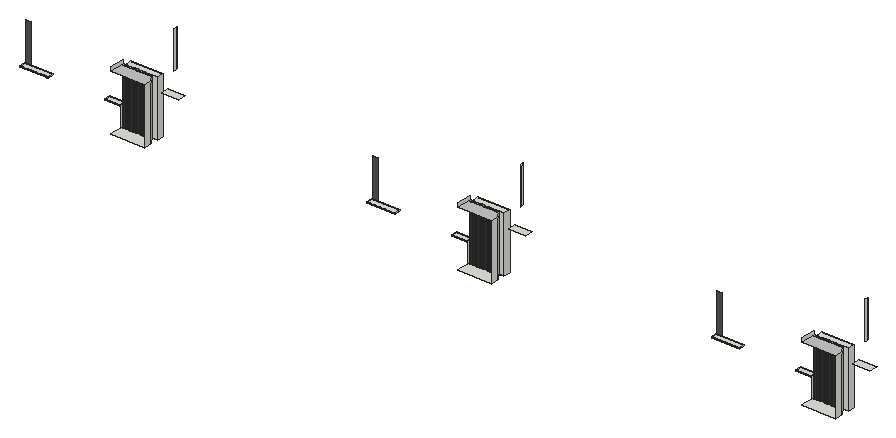
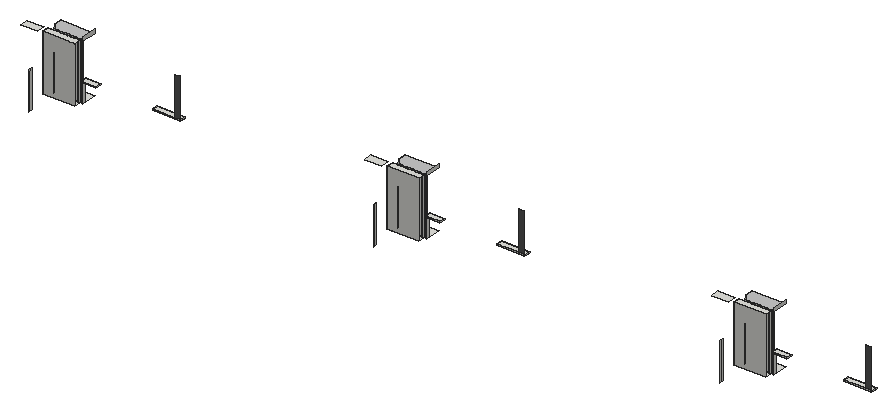
# SketchUp Ruby script. Lengths in inches.
U = 1.inch
M = Sketchup.active_model
def pt(a) = Geom::Point3d.new(a.map { |v| v * U })
def face(e, loops, mat)
  f = e.add_face(loops[0].map { |a| pt(a) })
  loops[1..].each { |l| e.add_face(l.map { |a| pt(a) }).erase! }
  f.material = f.back_material = mat if mat
  f
end
# faces: each face lists its corners as indices into pts; further lists are holes
def faces(e, pts, list, mat = nil) = list.each { |f| face(e, (f[0].is_a?(Array) ? f : [f]).map { |l| l.map { |i| pts[i] } }, mat) }
# xy, xz, yz: faces in a plane at the given z, y or x. An outline is a flat list of corners, or four numbers for a rectangle; further outlines are holes
def ring(l) = l.size == 4 ? [[l[0], l[1]], [l[2], l[1]], [l[2], l[3]], [l[0], l[3]]] : l.each_slice(2).to_a
def flat(e, list, mat, &to3) = list.each { |f| face(e, (f[0].is_a?(Array) ? f : [f]).map { |l| ring(l).map { |u, v| to3.(u, v) } }, mat) }
def xy(e, z, list, mat = nil) = flat(e, list, mat) { |x, y| [x, y, z] }
def xz(e, y, list, mat = nil) = flat(e, list, mat) { |x, z| [x, y, z] }
def yz(e, x, list, mat = nil) = flat(e, list, mat) { |y, z| [x, y, z] }
def lines(e, pts, list) = list.each { |a, b| e.add_line(pt(pts[a]), pt(pts[b])) }
# prism: a flat outline (further loops are holes) pulled along v
def prism(e, loops, v, mat = nil)
  f = face(e, loops, mat); d = Geom::Vector3d.new(v.map { |x| x * U })
  f.pushpull(f.normal.samedirection?(d) ? d.length : -d.length)
end
def box(e, o, s, mat = nil) = prism(e, [[o, [o[0] + s[0], o[1], o[2]], [o[0] + s[0], o[1] + s[1], o[2]], [o[0], o[1] + s[1], o[2]]]], [0, 0, s[2]], mat)
def at(x, y, z, deg = 0) = Geom::Transformation.translation(pt([x, y, z])) * Geom::Transformation.rotation(ORIGIN, Z_AXIS, deg.degrees)
def axes(o, x, y, z) = Geom::Transformation.new([*x, 0, *y, 0, *z, 0, *pt(o).to_a, 1])
def part(name) = M.definitions.add(name)
# library, detail: a bought-in or finely detailed component or shape, given as its bounding box
def library(name, o, s) = part(name).tap { |d| box(d.entities, o, s) }
def detail(e, o, s) = box(e.add_group.entities, o, s)
def put(e, d, t, mat = nil) = e.add_instance(d, t).tap { |i| i.material = mat if mat }
def group(e, t, mat = nil) = e.add_group.tap { |g| g.transformation = t; g.material = mat if mat }.entities
root = M.entities
M.materials.add("[Color M02]").color = [198, 198, 198]
M.materials.add("[Color M06]").color = [86, 86, 86]
M.materials.add("[Color M07]").color = [58, 58, 58]
xy(root,400.68,[[1098.03,273.0625,1175.84,273.0625,1175.84,289.5,1162.46,308.24,1162.46,304.93,1156.61,304.93,1156.61,308.24,1154.46,308.24,1154.46,304.93,1148.61,304.93,1148.61,308.24,1146.46,308.24,1146.46,304.93,1140.61,304.93,1140.61,308.24,1138.46,308.24,1138.46,304.93,1132.61,304.93,1132.61,308.24,1130.46,308.24,1130.46,304.93,1124.61,304.93,1124.61,308.24,1122.46,308.24,1122.46,304.93,1116.61,304.93,1116.61,308.24,1114.46,308.24,1114.46,304.93,1108.61,304.93,1108.61,308.24,1106.46,308.24,1106.46,304.93,1100.61,304.93,1100.61,308.24,1098.03,308.24],[1884.4,273.0625,1962.22,273.0625,1962.22,289.5,1948.83,308.24,1948.83,304.93,1942.98,304.93,1942.98,308.24,1940.83,308.24,1940.83,304.93,1934.98,304.93,1934.98,308.24,1932.83,308.24,1932.83,304.93,1926.98,304.93,1926.98,308.24,1924.83,308.24,1924.83,304.93,1918.98,304.93,1918.98,308.24,1916.83,308.24,1916.83,304.93,1910.98,304.93,1910.98,308.24,1908.83,308.24,1908.83,304.93,1902.98,304.93,1902.98,308.24,1900.83,308.24,1900.83,304.93,1894.98,304.93,1894.98,308.24,1892.83,308.24,1892.83,304.93,1886.98,304.93,1886.98,308.24,1884.4,308.24],[2664.78,273.0625,2742.59,273.0625,2742.59,289.5,2729.21,308.24,2729.21,304.93,2723.36,304.93,2723.36,308.24,2721.21,308.24,2721.21,304.93,2715.36,304.93,2715.36,308.24,2713.21,308.24,2713.21,304.93,2707.36,304.93,2707.36,308.24,2705.21,308.24,2705.21,304.93,2699.36,304.93,2699.36,308.24,2697.21,308.24,2697.21,304.93,2691.36,304.93,2691.36,308.24,2689.21,308.24,2689.21,304.93,2683.36,304.93,2683.36,308.24,2681.21,308.24,2681.21,304.93,2675.36,304.93,2675.36,308.24,2673.21,308.24,2673.21,304.93,2667.36,304.93,2667.36,308.24,2664.78,308.24],[1103.7,304.93,1106.46,308.24],[1108.61,304.93,1114.46,308.24],
  [1116.61,304.93,1122.46,308.24],[1124.61,304.93,1130.46,308.24],[1132.61,304.93,1138.46,308.24],[1140.61,304.93,1146.46,308.24],[1148.61,304.93,1154.46,308.24],
  [1156.61,304.93,1162.46,308.24],[1890.08,304.93,1892.83,308.24],[1894.98,304.93,1900.83,308.24],[1902.98,304.93,1908.83,308.24],[1910.98,304.93,1916.83,308.24],
  [1918.98,304.93,1924.83,308.24],[1926.98,304.93,1932.83,308.24],[1934.98,304.93,1940.83,308.24],[1942.98,304.93,1948.83,308.24],[2670.45,304.93,2673.21,308.24],
  [2675.36,304.93,2681.21,308.24],[2683.36,304.93,2689.21,308.24],[2691.36,304.93,2697.21,308.24],[2699.36,304.93,2705.21,308.24],[2707.36,304.93,2713.21,308.24],
  [2715.36,304.93,2721.21,308.24],[2723.36,304.93,2729.21,308.24],[1103.7,308.24,1175.84,323.81],[1890.08,308.24,1962.22,323.81],[2670.45,308.24,2742.59,323.81]])
xy(root,446.625,[[872.53,298.8125,936.06,301],[1064.56,298.8125,1098.03,301],[1658.9,298.8125,1722.43,301],[1850.93,298.8125,1884.4,301],[2439.28,298.8125,2502.81,301],
  [2631.31,298.8125,2664.78,301],[872.53,301,874.71,311.64],[874.71,301,933.87,311.64],[933.87,301,936.06,311.64],[1064.56,301,1066.62,311.64],
  [1066.62,301,1098.03,311.64],[1658.9,301,1661.09,311.64],[1661.09,301,1720.25,311.64],[1720.25,301,1722.43,311.64],[1850.93,301,1852.99,311.64],
  [1852.99,301,1884.4,311.64],[2439.28,301,2441.46,311.64],[2441.46,301,2500.62,311.64],[2500.62,301,2502.81,311.64],[2631.31,301,2633.37,311.64],
  [2633.37,301,2664.78,311.64]])
xy(root,449.125,[[872.53,298.8125,936.06,311.64],[1064.56,298.8125,1098.03,311.64],[1658.9,298.8125,1722.43,311.64],[1850.93,298.8125,1884.4,311.64],[2439.28,298.8125,2502.81,311.64],
  [2631.31,298.8125,2664.78,311.64]])
xy(root,512.23,[[1200.15,289.5,1239.03,308.24],[1986.53,289.5,2025.4,308.24],[2766.9,289.5,2805.78,308.24]])
xy(root,528.11,[[1103.7,304.93,1106.46,308.24],[1108.61,304.93,1114.46,308.24],[1116.61,304.93,1122.46,308.24],[1124.61,304.93,1130.46,308.24],[1132.61,304.93,1138.46,308.24],
  [1140.61,304.93,1146.46,308.24],[1148.61,304.93,1154.46,308.24],[1156.61,304.93,1162.46,308.24],[1890.08,304.93,1892.83,308.24],[1894.98,304.93,1900.83,308.24],
  [1902.98,304.93,1908.83,308.24],[1910.98,304.93,1916.83,308.24],[1918.98,304.93,1924.83,308.24],[1926.98,304.93,1932.83,308.24],[1934.98,304.93,1940.83,308.24],
  [1942.98,304.93,1948.83,308.24],[2670.45,304.93,2673.21,308.24],[2675.36,304.93,2681.21,308.24],[2683.36,304.93,2689.21,308.24],[2691.36,304.93,2697.21,308.24],
  [2699.36,304.93,2705.21,308.24],[2707.36,304.93,2713.21,308.24],[2715.36,304.93,2721.21,308.24],[2723.36,304.93,2729.21,308.24],[1103.7,308.24,1175.84,323.81],
  [1890.08,308.24,1962.22,323.81],[2670.45,308.24,2742.59,323.81]])
xy(root,528.11,[[1098.03,273.0625,1098.03,308.24,1100.61,308.24,1100.61,304.93,1106.46,304.93,1106.46,308.24,1108.61,308.24,1108.61,304.93,1114.46,304.93,1114.46,308.24,1116.61,308.24,1116.61,304.93,1122.46,304.93,1122.46,308.24,1124.61,308.24,1124.61,304.93,1130.46,304.93,1130.46,308.24,1132.61,308.24,1132.61,304.93,1138.46,304.93,1138.46,308.24,1140.61,308.24,1140.61,304.93,1146.46,304.93,1146.46,308.24,1148.61,308.24,1148.61,304.93,1154.46,304.93,1154.46,308.24,1156.61,308.24,1156.61,304.93,1162.46,304.93,1162.46,308.24,1175.84,289.5,1175.84,273.0625],[1884.4,273.0625,1884.4,308.24,1886.98,308.24,1886.98,304.93,1892.83,304.93,1892.83,308.24,1894.98,308.24,1894.98,304.93,1900.83,304.93,1900.83,308.24,1902.98,308.24,1902.98,304.93,1908.83,304.93,1908.83,308.24,1910.98,308.24,1910.98,304.93,1916.83,304.93,1916.83,308.24,1918.98,308.24,1918.98,304.93,1924.83,304.93,1924.83,308.24,1926.98,308.24,1926.98,304.93,1932.83,304.93,1932.83,308.24,1934.98,308.24,1934.98,304.93,1940.83,304.93,1940.83,308.24,1942.98,308.24,1942.98,304.93,1948.83,304.93,1948.83,308.24,1962.22,289.5,1962.22,273.0625],[2664.78,273.0625,2664.78,308.24,2667.36,308.24,2667.36,304.93,2673.21,304.93,2673.21,308.24,2675.36,308.24,2675.36,304.93,2681.21,304.93,2681.21,308.24,2683.36,308.24,2683.36,304.93,2689.21,304.93,2689.21,308.24,2691.36,308.24,2691.36,304.93,2697.21,304.93,2697.21,308.24,2699.36,308.24,2699.36,304.93,2705.21,304.93,2705.21,308.24,2707.36,308.24,2707.36,304.93,2713.21,304.93,2713.21,308.24,2715.36,308.24,2715.36,304.93,2721.21,304.93,2721.21,308.24,2723.36,308.24,2723.36,304.93,2729.21,304.93,2729.21,308.24,2742.59,289.5,2742.59,273.0625]],"[Color M02]")
xz(root,298.8125,[[872.53,446.625,936.06,449.125],[1064.56,446.625,1098.03,449.125],[1658.9,446.625,1722.43,449.125],[1850.93,446.625,1884.4,449.125],[2439.28,446.625,2502.81,449.125],
  [2631.31,446.625,2664.78,449.125]])
xz(root,304.93,[[1100.61,400.68,1106.46,528.11],[1108.61,400.68,1114.46,528.11],[1116.61,400.68,1122.46,528.11],[1124.61,400.68,1130.46,528.11],[1132.61,400.68,1138.46,528.11],
  [1140.61,400.68,1146.46,528.11],[1148.61,400.68,1154.46,528.11],[1156.61,400.68,1162.46,528.11],[1886.98,400.68,1892.83,528.11],[1894.98,400.68,1900.83,528.11],
  [1902.98,400.68,1908.83,528.11],[1910.98,400.68,1916.83,528.11],[1918.98,400.68,1924.83,528.11],[1926.98,400.68,1932.83,528.11],[1934.98,400.68,1940.83,528.11],
  [1942.98,400.68,1948.83,528.11],[2667.36,400.68,2673.21,528.11],[2675.36,400.68,2681.21,528.11],[2683.36,400.68,2689.21,528.11],[2691.36,400.68,2697.21,528.11],
  [2699.36,400.68,2705.21,528.11],[2707.36,400.68,2713.21,528.11],[2715.36,400.68,2721.21,528.11],[2723.36,400.68,2729.21,528.11]],"[Color M07]")
xz(root,308.24,[[1162.46,400.68,1175.84,528.11],[1948.83,400.68,1962.22,528.11],[2729.21,400.68,2742.59,528.11]])
xz(root,308.24,[[1098.03,400.68,1100.61,528.11],[1106.46,400.68,1108.61,528.11],[1114.46,400.68,1116.61,528.11],[1122.46,400.68,1124.61,528.11],[1130.46,400.68,1132.61,528.11],
  [1138.46,400.68,1140.61,528.11],[1146.46,400.68,1148.61,528.11],[1154.46,400.68,1156.61,528.11],[1884.4,400.68,1886.98,528.11],[1892.83,400.68,1894.98,528.11],
  [1900.83,400.68,1902.98,528.11],[1908.83,400.68,1910.98,528.11],[1916.83,400.68,1918.98,528.11],[1924.83,400.68,1926.98,528.11],[1932.83,400.68,1934.98,528.11],
  [1940.83,400.68,1942.98,528.11],[2664.78,400.68,2667.36,528.11],[2673.21,400.68,2675.36,528.11],[2681.21,400.68,2683.36,528.11],[2689.21,400.68,2691.36,528.11],
  [2697.21,400.68,2699.36,528.11],[2705.21,400.68,2707.36,528.11],[2713.21,400.68,2715.36,528.11],[2721.21,400.68,2723.36,528.11]],"[Color M07]")
xz(root,311.64,[[872.53,446.625,874.71,449.125],[874.71,446.625,885.36,449.125],[885.36,446.625,936.06,449.125],[1064.56,446.625,1087.38,449.125],[1087.38,446.625,1098.03,449.125],
  [1658.9,446.625,1661.09,449.125],[1661.09,446.625,1671.73,449.125],[1671.73,446.625,1722.43,449.125],[1850.93,446.625,1873.76,449.125],[1873.76,446.625,1884.4,449.125],
  [2439.28,446.625,2441.46,449.125],[2441.46,446.625,2452.11,449.125],[2452.11,446.625,2502.81,449.125],[2631.31,446.625,2654.13,449.125],[2654.13,446.625,2664.78,449.125]])
xz(root,311.64,[[874.71,449.125,885.36,536.4375],[1661.09,449.125,1671.73,536.4375],[2441.46,449.125,2452.11,536.4375]],"[Color M06]")
xz(root,323.81,[[1103.7,400.68,1175.84,528.11],[1890.08,400.68,1962.22,528.11],[2670.45,400.68,2742.59,528.11]])
yz(root,872.53,[[298.8125,446.625,311.64,449.125]])
yz(root,936.06,[[298.8125,446.625,311.64,449.125]])
yz(root,1064.56,[[298.8125,446.625,311.64,449.125]])
yz(root,1098.03,[[301,400.68,308.24,446.625],[298.8125,446.625,308.24,449.125],[308.24,446.625,311.64,449.125],[452.5625,451.1875,456.375,536.4375],[456.375,451.1875,459.0625,536.4375],
  [273.0625,528.11,308.24,536.4375]])
yz(root,1100.61,[[304.93,400.68,308.24,528.11]])
yz(root,1106.46,[[304.93,400.68,308.24,528.11]])
yz(root,1108.61,[[304.93,400.68,308.24,528.11]])
yz(root,1114.46,[[304.93,400.68,308.24,528.11]])
yz(root,1116.61,[[304.93,400.68,308.24,528.11]])
yz(root,1122.46,[[304.93,400.68,308.24,528.11]])
yz(root,1124.61,[[304.93,400.68,308.24,528.11]])
yz(root,1130.46,[[304.93,400.68,308.24,528.11]])
yz(root,1132.61,[[304.93,400.68,308.24,528.11]])
yz(root,1138.46,[[304.93,400.68,308.24,528.11]])
yz(root,1140.61,[[304.93,400.68,308.24,528.11]])
yz(root,1146.46,[[304.93,400.68,308.24,528.11]])
yz(root,1148.61,[[304.93,400.68,308.24,528.11]])
yz(root,1154.46,[[304.93,400.68,308.24,528.11]])
yz(root,1156.61,[[304.93,400.68,308.24,528.11]])
yz(root,1162.46,[[304.93,400.68,308.24,528.11]])
yz(root,1175.84,[[273.0625,400.68,289.5,528.11],[308.24,400.68,323.81,528.11]])
yz(root,1658.9,[[298.8125,446.625,311.64,449.125]])
yz(root,1722.43,[[298.8125,446.625,311.64,449.125]])
yz(root,1850.93,[[298.8125,446.625,311.64,449.125]])
yz(root,1884.4,[[301,400.68,308.24,446.625],[298.8125,446.625,308.24,449.125],[308.24,446.625,311.64,449.125],[452.5625,451.1875,456.375,536.4375],[456.375,451.1875,459.0625,536.4375],
  [273.0625,528.11,308.24,536.4375]])
yz(root,1886.98,[[304.93,400.68,308.24,528.11]])
yz(root,1892.83,[[304.93,400.68,308.24,528.11]])
yz(root,1894.98,[[304.93,400.68,308.24,528.11]])
yz(root,1900.83,[[304.93,400.68,308.24,528.11]])
yz(root,1902.98,[[304.93,400.68,308.24,528.11]])
yz(root,1908.83,[[304.93,400.68,308.24,528.11]])
yz(root,1910.98,[[304.93,400.68,308.24,528.11]])
yz(root,1916.83,[[304.93,400.68,308.24,528.11]])
yz(root,1918.98,[[304.93,400.68,308.24,528.11]])
yz(root,1924.83,[[304.93,400.68,308.24,528.11]])
yz(root,1926.98,[[304.93,400.68,308.24,528.11]])
yz(root,1932.83,[[304.93,400.68,308.24,528.11]])
yz(root,1934.98,[[304.93,400.68,308.24,528.11]])
yz(root,1940.83,[[304.93,400.68,308.24,528.11]])
yz(root,1942.98,[[304.93,400.68,308.24,528.11]])
yz(root,1948.83,[[304.93,400.68,308.24,528.11]])
yz(root,1962.22,[[273.0625,400.68,289.5,528.11],[308.24,400.68,323.81,528.11]])
yz(root,2439.28,[[298.8125,446.625,311.64,449.125]])
yz(root,2502.81,[[298.8125,446.625,311.64,449.125]])
yz(root,2631.31,[[298.8125,446.625,311.64,449.125]])
yz(root,2664.78,[[301,400.68,308.24,446.625],[298.8125,446.625,308.24,449.125],[308.24,446.625,311.64,449.125],[452.5625,451.1875,456.375,536.4375],[456.375,451.1875,459.0625,536.4375],
  [273.0625,528.11,308.24,536.4375]])
yz(root,2667.36,[[304.93,400.68,308.24,528.11]])
yz(root,2673.21,[[304.93,400.68,308.24,528.11]])
yz(root,2675.36,[[304.93,400.68,308.24,528.11]])
yz(root,2681.21,[[304.93,400.68,308.24,528.11]])
yz(root,2683.36,[[304.93,400.68,308.24,528.11]])
yz(root,2689.21,[[304.93,400.68,308.24,528.11]])
yz(root,2691.36,[[304.93,400.68,308.24,528.11]])
yz(root,2697.21,[[304.93,400.68,308.24,528.11]])
yz(root,2699.36,[[304.93,400.68,308.24,528.11]])
yz(root,2705.21,[[304.93,400.68,308.24,528.11]])
yz(root,2707.36,[[304.93,400.68,308.24,528.11]])
yz(root,2713.21,[[304.93,400.68,308.24,528.11]])
yz(root,2715.36,[[304.93,400.68,308.24,528.11]])
yz(root,2721.21,[[304.93,400.68,308.24,528.11]])
yz(root,2723.36,[[304.93,400.68,308.24,528.11]])
yz(root,2729.21,[[304.93,400.68,308.24,528.11]])
yz(root,2742.59,[[273.0625,400.68,289.5,528.11],[308.24,400.68,323.81,528.11]])
p = [[1175.84,289.5,528.11],[1162.46,308.24,528.11],[1162.46,308.24,400.68],[1175.84,289.5,400.68],[1962.22,289.5,528.11],[1948.83,308.24,528.11],
  [1948.83,308.24,400.68],[1962.22,289.5,400.68],[2742.59,289.5,528.11],[2729.21,308.24,528.11],[2729.21,308.24,400.68],[2742.59,289.5,400.68]]
faces(root,p,[[0,1,2,3],[4,5,6,7],[8,9,10,11]])
